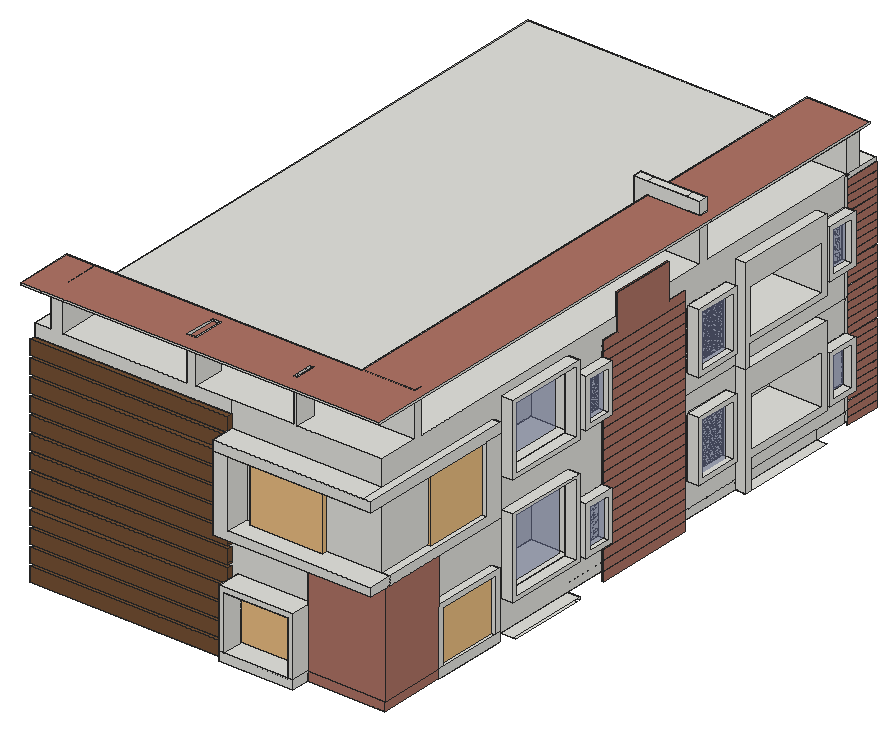
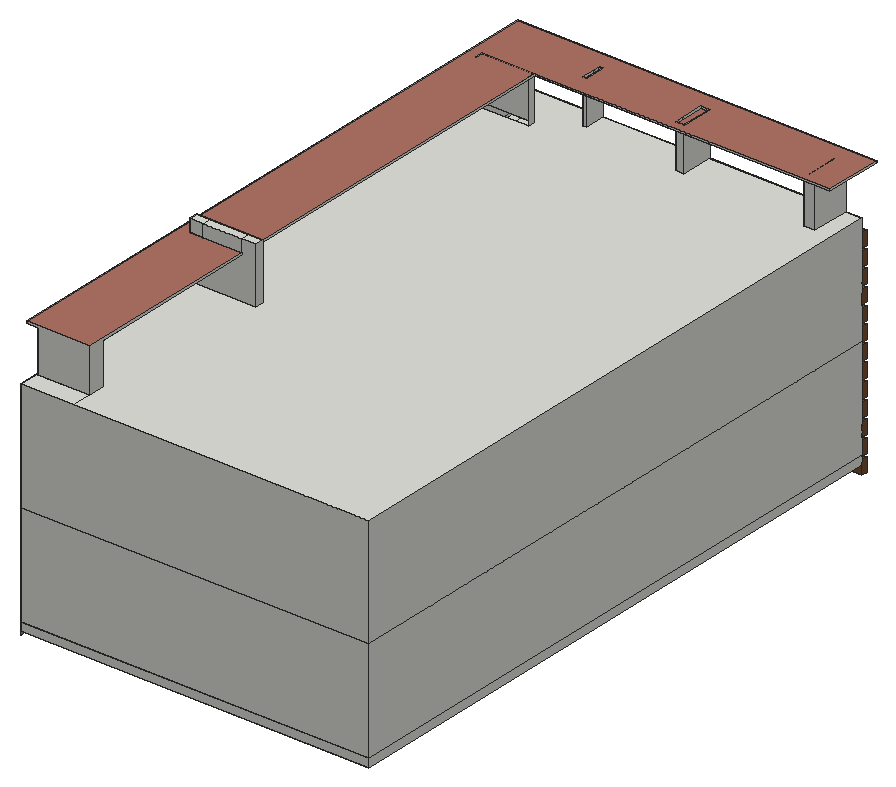
# SketchUp Ruby script. Lengths in inches.
U = 1.inch
M = Sketchup.active_model
def pt(a) = Geom::Point3d.new(a.map { |v| v * U })
def face(e, loops, mat)
  f = e.add_face(loops[0].map { |a| pt(a) })
  loops[1..].each { |l| e.add_face(l.map { |a| pt(a) }).erase! }
  f.material = f.back_material = mat if mat
  f
end
# faces: each face lists its corners as indices into pts; further lists are holes
def faces(e, pts, list, mat = nil) = list.each { |f| face(e, (f[0].is_a?(Array) ? f : [f]).map { |l| l.map { |i| pts[i] } }, mat) }
# xy, xz, yz: faces in a plane at the given z, y or x. An outline is a flat list of corners, or four numbers for a rectangle; further outlines are holes
def ring(l) = l.size == 4 ? [[l[0], l[1]], [l[2], l[1]], [l[2], l[3]], [l[0], l[3]]] : l.each_slice(2).to_a
def flat(e, list, mat, &to3) = list.each { |f| face(e, (f[0].is_a?(Array) ? f : [f]).map { |l| ring(l).map { |u, v| to3.(u, v) } }, mat) }
def xy(e, z, list, mat = nil) = flat(e, list, mat) { |x, y| [x, y, z] }
def xz(e, y, list, mat = nil) = flat(e, list, mat) { |x, z| [x, y, z] }
def yz(e, x, list, mat = nil) = flat(e, list, mat) { |y, z| [x, y, z] }
def lines(e, pts, list) = list.each { |a, b| e.add_line(pt(pts[a]), pt(pts[b])) }
# prism: a flat outline (further loops are holes) pulled along v
def prism(e, loops, v, mat = nil)
  f = face(e, loops, mat); d = Geom::Vector3d.new(v.map { |x| x * U })
  f.pushpull(f.normal.samedirection?(d) ? d.length : -d.length)
end
def box(e, o, s, mat = nil) = prism(e, [[o, [o[0] + s[0], o[1], o[2]], [o[0] + s[0], o[1] + s[1], o[2]], [o[0], o[1] + s[1], o[2]]]], [0, 0, s[2]], mat)
def at(x, y, z, deg = 0) = Geom::Transformation.translation(pt([x, y, z])) * Geom::Transformation.rotation(ORIGIN, Z_AXIS, deg.degrees)
def axes(o, x, y, z) = Geom::Transformation.new([*x, 0, *y, 0, *z, 0, *pt(o).to_a, 1])
def part(name) = M.definitions.add(name)
# library, detail: a bought-in or finely detailed component or shape, given as its bounding box
def library(name, o, s) = part(name).tap { |d| box(d.entities, o, s) }
def detail(e, o, s) = box(e.add_group.entities, o, s)
def put(e, d, t, mat = nil) = e.add_instance(d, t).tap { |i| i.material = mat if mat }
def group(e, t, mat = nil) = e.add_group.tap { |g| g.transformation = t; g.material = mat if mat }.entities
root = M.entities
M.materials.add("Artistic-Tile__Vetromarmi__Granada-Smoke-Glass-and-Stone-Wat").color = [172, 173, 170]
M.materials.add("[Sandstone]").color = [118, 81, 52]
M.materials.add("[Stone Flagstone Ashlar]").color = [175, 116, 102]
M.materials.add("[Translucent Glass Sky Reflection]").color = [126, 138, 183]
M.materials["[Translucent Glass Sky Reflection]"].alpha = 0.52
c1 = part("Group\#12")
prism(c1.entities,[[[0,67.07,0],[0,0,0],[0,0,12.125],[0,67.07,12.125],[0,139.8125,12.125],[0,139.8125,0]]],[2.5,0,0])
c2 = part("Group\#11")
prism(c2.entities,[[[271.64,0,19.53],[271.64,0,2.36],[271.64,0,0],[0,0,0],[0,0,19.53]]],[0,-6.9375,0])
c3 = part("Group\#13")
box(c3.entities,[0,0,0],[1.1875,48.5625,8.8125])
c4 = library("AS-120-mm\#2",[0,0,0],[88.21,4.72,72.97])
c5 = part("Group\#6")
xy(c5.entities,0,[[[0,0,45,67.3125],[6.42,6.42,38.58,60.9]],[6.42,6.42,38.58,60.9]])
xy(c5.entities,14.3125,[[[0,0,45,67.3125],[6.42,6.42,38.58,60.9]]])
xz(c5.entities,0,[[0,0,45,14.3125]])
xz(c5.entities,6.42,[[6.42,0,38.58,14.3125]])
xz(c5.entities,60.9,[[6.42,0,38.58,14.3125]])
xz(c5.entities,67.3125,[[0,0,45,14.3125]])
yz(c5.entities,0,[[0,0,67.3125,14.3125]])
yz(c5.entities,6.42,[[6.42,0,60.9,14.3125]])
yz(c5.entities,38.58,[[6.42,0,60.9,14.3125]])
yz(c5.entities,45,[[0,0,67.3125,14.3125]])
c6 = part("Group\#5")
xy(c6.entities,0,[[[0,0,66.75,83.5625],[5.83,5.83,60.92,77.73]],[5.83,5.83,60.92,77.73]])
xy(c6.entities,15.625,[[[0,0,66.75,83.5625],[5.83,5.83,60.92,77.73]]])
xz(c6.entities,0,[[0,0,66.75,15.625]])
xz(c6.entities,5.83,[[5.83,0,60.92,15.625]])
xz(c6.entities,77.73,[[5.83,0,60.92,15.625]])
xz(c6.entities,83.5625,[[0,0,66.75,15.625]])
yz(c6.entities,0,[[0,0,83.5625,15.625]])
yz(c6.entities,5.83,[[5.83,0,77.73,15.625]])
yz(c6.entities,60.92,[[5.83,0,77.73,15.625]])
yz(c6.entities,66.75,[[0,0,83.5625,15.625]])
c7 = part("Artistic-Tile__Vetromarmi__Granada-Smoke-Glass-and-Stone-Wat")
xy(c7.entities,0,[[0,0,24,24]],"[Translucent Glass Sky Reflection]")
c8 = library("AS-120-mm\#4",[0,0,0],[101.61,4.72,91.97])
c9 = library("AS-120-mm\#5",[0,0,0],[88.21,4.72,91.97])
xy(root,440.43,[[763.75,300.49,763.75,409.52,814.625,409.52,814.625,404.56,831,404.56,831,300.49]])
xy(root,443.8125,[[814.625,697.51,829.375,705.8]])
xy(root,444.1875,[[616.81,57.85,623.61,90.47],[623.61,57.85,711.82,90.47],[711.82,57.85,718.625,90.47],[718.69,83.16,814.625,83.16,814.625,174.47,824.98,174.47,824.98,181.28,814.625,181.28,814.625,271.67,824.98,271.67,824.98,278.47,814.625,278.47,814.625,939.04,336.5625,939.04,336.5625,90.47,718.69,90.47],[718.625,83.16,718.69,90.47],
  [814.625,83.16,824.98,174.47],[824.98,174.47,825.8125,181.28],[814.625,181.28,825.8125,271.67],[824.98,271.67,825.8125,278.47],[814.625,295.05,831,409.52],
  [814.625,697.51,828.9375,837.09]])
xy(root,456.1875,[[616.81,57.85,623.61,90.47],[623.61,57.85,711.82,90.47],[711.82,57.85,718.625,90.47],[718.69,83.16,718.69,90.47,336.5625,90.47,336.5625,939.04,814.625,939.04,814.625,409.52,763.75,409.52,763.75,295.05,814.625,295.05,814.625,278.47,825.8125,278.47,825.8125,271.67,814.625,271.67,814.625,181.28,825.8125,181.28,825.8125,174.47,814.625,174.47,814.625,83.16],[718.625,83.16,718.69,90.47],
  [814.625,83.16,824.98,174.47],[824.98,83.16,825.8125,174.47],[814.625,181.28,825.8125,271.67]])
xy(root,484.82,[[814.625,705.8,829.375,837.09]])
xy(root,487.375,[[814.625,295.05,831,409.52]])
xy(root,491.4375,[[763.75,295.05,814.625,300.49],[763.75,300.49,814.625,409.52],[814.625,300.49,831,404.56]])
xy(root,494.39,[[757.625,707.08,829.375,827.53]])
xy(root,528.43,[[814.625,181.28,825.8125,271.67]])
xy(root,531.09,[[623.61,57.85,711.82,90.47]])
xy(root,535.23,[[814.625,174.47,825.8125,278.47]])
xy(root,537.9,[[616.81,57.85,718.625,90.47]])
xy(root,562.5,[[757.625,707.08,829.375,827.53]])
xy(root,592.89,[[763.75,300.49,763.75,409.52,814.625,409.52,814.625,404.56,831,404.56,831,300.49]])
xy(root,596.25,[[814.625,295.05,831,409.52],[814.625,697.51,829.375,837.09]])
xy(root,596.375,[[763.75,295.05,814.625,409.52],[814.625,697.51,828.9375,704.26]])
xy(root,608.25,[[628.73,57.85,825.8125,90.47],[814.625,90.64,825.8125,257.14]])
xy(root,626.2,[[814.625,704.26,828.9375,837.09]])
xy(root,634.0625,[[755.875,705.37,828.9375,829.23]])
xy(root,638,[[814.625,295.05,831,409.52]])
xy(root,643.1875,[[763.75,295.05,814.625,300.49],[763.75,300.49,814.625,409.52],[814.625,300.49,831,404.56]])
xy(root,695.82,[[755.875,705.37,828.9375,829.23]])
xy(root,700.22,[[628.73,57.85,814.625,90.47],[814.625,57.85,825.8125,257.14]])
xy(root,713.98,[[608.2,57.85,814.625,90.47],[814.625,57.85,825.8125,280.55]])
xy(root,728.06,[[814.625,697.51,828.9375,837.09]])
xy(root,731.48,[[763.75,300.49,763.75,409.52,814.625,409.52,814.625,404.56,831,404.56,831,300.49]])
xy(root,735.98,[[814.625,295.05,831,409.52]])
xy(root,742.93,[[814.625,890.48,815.8125,939.04]])
xy(root,748.3125,[[336.5625,90.47,359.68,90.47,359.68,142.97,375.49,142.97,375.49,90.47,546.88,90.47,546.88,133.72,558.94,133.72,558.94,90.47,693.12,90.47,693.12,118.97,697.99,118.97,697.99,90.47,814.625,90.47,814.625,146.875,742.8125,146.875,742.8125,156.625,814.625,156.625,814.625,637.28,723.375,637.28,723.375,649.15,814.625,649.15,814.625,889.53,742.61,889.53,742.61,939.04,336.5625,939.04],[814.625,886.91,817.0625,890.48],[742.61,889.53,814.625,911.1],[814.625,890.48,815.8125,911.1],[742.61,911.1,815.8125,939.04]])
xy(root,805.9375,[[742.61,637.28,796.05,649.15],[814.625,637.28,814.625,649.15,742.61,649.15,742.61,889.53,829.6875,889.53,829.6875,637.28],[814.625,889.53,829.6875,911.1]])
xy(root,805.9375,[[336.5625,66.4,336.5625,145.68,742.61,145.68,742.61,637.28,829.6875,637.28,829.6875,66.4]],"[Stone Flagstone Ashlar]")
xy(root,807.1875,[[359.68,90.47,375.49,142.97]])
xy(root,808.4375,[[742.61,146.875,742.8125,156.625]])
xy(root,808.4375,[[[336.5625,66.4,829.6875,66.4,829.6875,911.1,742.61,911.1,742.61,156.625,742.8125,156.625,742.8125,146.875,742.61,146.875,742.61,145.68,336.5625,145.68],[546.88,90.47,558.94,133.72],[796.05,637.28,814.625,649.15],[693.12,90.47,697.99,118.97]]],"[Stone Flagstone Ashlar]")
xy(root,825.5625,[[723.375,637.28,742.61,649.15],[742.61,637.28,796.05,649.15],[796.05,637.28,814.625,649.15]])
xz(root,57.85,[[616.81,444.1875,718.625,456.1875],[616.81,456.1875,623.61,456.1875,623.61,531.09,711.82,531.09,711.82,456.1875,718.625,456.1875,718.625,537.9,616.81,537.9],[608.2,596.375,825.8125,596.375,825.8125,608.25,628.73,608.25,628.73,700.22,608.2,700.22],[608.2,700.22,825.8125,713.98]])
xz(root,66.4,[[336.5625,805.9375,829.6875,808.4375]])
xz(root,83.16,[[718.625,444.1875,718.69,456.1875]])
xz(root,83.16,[[718.69,444.1875,824.98,456.1875],[718.625,456.1875,825.8125,596.25]],"[Stone Flagstone Ashlar]")
xz(root,90.47,[[608.2,444.1875,616.81,456.1875],[718.625,444.1875,718.69,456.1875],[336.5625,456.1875,616.81,456.1875,616.81,537.9,718.625,537.9,718.625,596.25,336.5625,596.25],[623.61,456.1875,711.82,531.09],[336.5625,596.375,608.2,711.62],
  [814.625,596.375,825.8125,608.25],[628.73,608.25,814.625,700.22],[608.2,713.98,814.625,713.98,814.625,748.3125,697.99,748.3125,697.99,808.4375,693.12,808.4375,693.12,748.3125,608.2,748.3125],[336.5625,731.15,608.2,731.15,608.2,748.3125,558.94,748.3125,558.94,808.4375,546.88,808.4375,546.88,748.3125,375.49,748.3125,375.49,807.1875,359.68,807.1875,359.68,748.3125,336.5625,748.3125]])
xz(root,90.64,[[814.625,596.375,825.8125,608.25]])
xz(root,118.97,[[693.12,748.3125,697.99,808.4375]])
xz(root,133.72,[[546.88,748.3125,558.94,808.4375]])
xz(root,142.97,[[359.68,748.3125,375.49,807.1875]])
xz(root,145.68,[[336.5625,805.9375,742.61,808.4375]])
xz(root,146.875,[[742.8125,748.3125,814.625,808.4375]])
xz(root,174.47,[[824.98,444.1875,825.8125,456.1875],[814.625,535.23,825.8125,596.25]])
xz(root,181.28,[[814.625,456.1875,825.8125,528.43]])
xz(root,257.14,[[814.625,608.25,825.8125,700.22]])
xz(root,271.67,[[814.625,456.1875,825.8125,528.43]])
xz(root,278.47,[[814.625,444.1875,825.8125,456.1875],[814.625,456.1875,825.8125,535.23]])
xz(root,280.55,[[814.625,596.375,825.8125,700.22],[814.625,700.22,825.8125,713.98]])
xz(root,295.05,[[814.625,487.375,831,596.25],[763.75,596.25,814.625,596.375],[814.625,638,831,735.98]])
xz(root,300.49,[[763.75,491.4375,831,592.89],[763.75,643.1875,831,731.48]])
xz(root,404.56,[[814.625,491.4375,831,592.89],[814.625,643.1875,831,731.48]])
xz(root,409.52,[[763.75,440.43,814.625,444.1875],[814.625,440.43,831,444.1875],[814.625,487.375,831,592.89],[763.75,491.4375,814.625,592.89],[763.75,592.89,814.625,596.25],
  [814.625,592.89,831,596.25],[763.75,596.25,814.625,596.375],[814.625,638,831,731.48],[763.75,643.1875,814.625,731.48],[763.75,731.48,814.625,735.98],
  [814.625,731.48,831,735.98]])
xz(root,637.28,[[723.375,748.3125,814.625,748.3125,814.625,805.9375,796.05,805.9375,796.05,808.4375,814.625,808.4375,814.625,825.5625,723.375,825.5625],[796.05,805.9375,814.625,808.4375]])
xz(root,649.15,[[723.375,748.3125,723.375,825.5625,742.61,825.5625,742.61,805.9375,814.625,805.9375,814.625,748.3125],[742.61,805.9375,796.05,825.5625],[796.05,805.9375,814.625,808.4375],[796.05,808.4375,814.625,825.5625]])
xz(root,697.51,[[814.625,443.8125,828.9375,444.1875],[828.9375,443.8125,829.375,443.8125,829.375,596.25,814.625,596.25,814.625,444.1875,828.9375,444.1875],[814.625,596.375,828.9375,728.06]])
xz(root,704.26,[[814.625,596.375,828.9375,626.2]])
xz(root,705.37,[[755.875,634.0625,828.9375,695.82]])
xz(root,705.8,[[814.625,443.8125,829.375,484.82]])
xz(root,707.08,[[757.625,494.39,829.375,562.5]])
xz(root,827.53,[[757.625,494.39,829.375,562.5]])
xz(root,829.23,[[755.875,634.0625,828.9375,695.82]])
xz(root,837.09,[[814.625,484.82,829.375,596.25],[814.625,626.2,828.9375,728.06]])
xz(root,889.53,[[742.61,748.3125,814.625,805.9375]])
xz(root,890.48,[[814.625,742.93,815.8125,748.3125]])
xz(root,911.1,[[742.61,748.3125,742.61,808.4375,829.6875,808.4375,829.6875,805.9375,814.625,805.9375,814.625,748.3125]])
xz(root,939.04,[[336.5625,456.1875,814.625,596.25],[336.5625,596.375,814.625,748.3125],[814.625,742.93,815.8125,748.3125]])
yz(root,336.5625,[[90.47,456.1875,939.04,596.25],[90.47,596.375,939.04,748.3125],[66.4,805.9375,145.68,808.4375]])
yz(root,359.68,[[90.47,748.3125,142.97,807.1875]])
yz(root,375.49,[[90.47,748.3125,142.97,807.1875]])
yz(root,546.88,[[90.47,748.3125,133.72,808.4375]])
yz(root,558.94,[[90.47,748.3125,133.72,808.4375]])
yz(root,608.2,[[57.85,596.375,90.47,700.22],[57.85,700.22,90.47,713.98]])
yz(root,616.81,[[57.85,444.1875,90.47,456.1875],[57.85,456.1875,90.47,537.9]])
yz(root,623.61,[[57.85,456.1875,90.47,531.09]])
yz(root,628.73,[[57.85,608.25,90.47,700.22]])
yz(root,693.12,[[90.47,748.3125,118.97,808.4375]])
yz(root,697.99,[[90.47,748.3125,118.97,808.4375]])
yz(root,711.82,[[57.85,456.1875,90.47,531.09]])
yz(root,718.625,[[57.85,444.1875,83.16,456.1875],[83.16,444.1875,90.47,456.1875],[57.85,456.1875,83.16,537.9],[83.16,537.9,90.47,596.25]])
yz(root,718.69,[[83.16,444.1875,90.47,456.1875]])
yz(root,723.375,[[637.28,748.3125,649.15,825.5625]])
yz(root,742.61,[[889.53,748.3125,889.53,805.9375,649.15,805.9375,649.15,808.4375,911.1,808.4375,911.1,748.3125],[145.68,805.9375,637.28,808.4375],[637.28,805.9375,649.15,808.4375]])
yz(root,742.8125,[[146.875,748.3125,156.625,808.4375]])
yz(root,755.875,[[705.37,634.0625,829.23,695.82]])
yz(root,757.625,[[707.08,494.39,827.53,562.5]])
yz(root,763.75,[[295.05,456.1875,409.52,491.4375],[300.49,491.4375,409.52,592.89],[295.05,596.25,409.52,596.375],[295.05,596.375,409.52,643.1875],[300.49,643.1875,409.52,731.48]])
yz(root,796.05,[[637.28,805.9375,649.15,808.4375]])
yz(root,814.625,[[697.51,443.8125,705.8,444.1875],[[278.47,444.1875,468.48,444.1875,468.48,728.58,535.54,728.58,535.54,748.3125,156.625,748.3125,156.625,808.4375,146.875,808.4375,146.875,748.3125,90.47,748.3125,90.47,713.98,280.55,713.98,280.55,596.25,174.47,596.25,174.47,535.23,278.47,535.23],[295.05,487.375,409.52,596.375],[295.05,638,409.52,735.98]],[468.48,444.1875,535.54,456.1875],[535.54,444.1875,697.51,456.1875],[697.51,444.1875,705.8,456.1875],
  [705.8,444.1875,837.09,456.1875],[886.91,444.1875,890.48,456.1875],[181.28,456.1875,271.67,528.43],[468.48,456.1875,535.54,596.25],[535.54,456.1875,697.51,596.25],
  [705.8,456.1875,886.91,456.1875,886.91,596.25,837.09,596.25,837.09,484.82,705.8,484.82],[886.91,456.1875,890.48,596.25],[890.48,456.1875,939.04,596.25],[295.05,487.375,409.52,491.4375],[404.56,491.4375,409.52,592.89],
  [295.05,596.25,409.52,596.375],[468.48,596.25,535.54,596.375],[535.54,596.25,697.51,596.375],[697.51,596.25,837.09,596.375],[886.91,596.25,890.48,596.375],
  [90.47,596.375,90.64,596.375,90.64,608.25,257.14,608.25,257.14,700.22,90.47,700.22],[468.48,596.375,535.54,716.46],[535.54,596.375,697.51,596.375,697.51,728.06,837.09,728.06,837.09,626.2,704.26,626.2,704.26,596.375,886.91,596.375,886.91,748.3125,649.15,748.3125,649.15,805.9375,637.28,805.9375,637.28,748.3125,535.54,748.3125,535.54,728.58,608.29,728.58,608.29,716.46,535.54,716.46],[886.91,596.375,890.48,748.3125],[890.48,596.375,939.04,733],
  [295.05,638,409.52,643.1875],[404.56,643.1875,409.52,731.48],[890.48,741.8125,939.04,742.93],[889.53,748.3125,911.1,805.9375],[637.28,805.9375,649.15,808.4375],
  [637.28,808.4375,649.15,825.5625]])
yz(root,815.8125,[[890.48,742.93,939.04,748.3125]])
yz(root,824.98,[[83.16,444.1875,174.47,456.1875]],"[Stone Flagstone Ashlar]")
yz(root,825.8125,[[174.47,444.1875,278.47,456.1875],[174.47,456.1875,181.28,456.1875,181.28,528.43,271.67,528.43,271.67,456.1875,278.47,456.1875,278.47,535.23,174.47,535.23],[57.85,596.375,90.47,608.25],[90.64,596.375,280.55,596.375,280.55,700.22,257.14,700.22,257.14,608.25,90.64,608.25],[57.85,700.22,280.55,713.98]])
yz(root,825.8125,[[83.16,456.1875,174.47,596.25]],"[Stone Flagstone Ashlar]")
yz(root,828.9375,[[697.51,596.375,704.26,596.375,704.26,626.2,837.09,626.2,837.09,718.19,705.37,718.19,705.37,695.82,829.23,695.82,829.23,634.0625,705.37,634.0625,705.37,718.19,837.09,718.19,837.09,728.06,697.51,728.06]])
yz(root,829.375,[[[697.51,443.8125,705.8,443.8125,705.8,484.82,837.09,484.82,837.09,596.25,697.51,596.25],[707.08,494.39,827.53,562.5]]])
yz(root,829.6875,[[66.4,805.9375,637.28,808.4375],[637.28,805.9375,911.1,808.4375]])
yz(root,831,[[[295.05,487.375,409.52,596.25],[300.49,491.4375,404.56,592.89]],[[295.05,638,409.52,735.98],[300.49,643.1875,404.56,731.48]]])
p = [[608.2,90.47,596.25],[608.2,90.47,596.375],[817.125,493.42,728.58],[814.625,493.42,728.58],[817.125,580.72,728.58],[814.625,580.72,728.58]]
lines(root,p,[[0,1],[2,3],[4,5]])
put(root,c1,at(814.625,468.48,431.64),"[Stone Flagstone Ashlar]")
put(root,c2,at(336.5625,90.47,431.87),"[Sandstone]")
put(root,c3,at(814.625,890.48,439.375),"[Stone Flagstone Ashlar]")
g1 = group(root,at(336.5625,690.47,444.1875))
box(g1,[0,-600,0],[478.0625,848.5625,12])
put(root,c1,at(814.625,468.48,445.21),"[Stone Flagstone Ashlar]")
put(root,c3,at(814.625,890.48,449.5),"[Stone Flagstone Ashlar]")
put(root,c2,at(336.5625,90.47,455.18),"[Sandstone]")
put(root,c4,at(815.4375,271.67,455.46,-90))
put(root,c4,at(623.61,85.95,458.12))
put(root,c1,at(814.625,468.48,458.77),"[Stone Flagstone Ashlar]")
put(root,c3,at(814.625,890.48,459.625),"[Stone Flagstone Ashlar]")
put(root,c3,at(814.625,890.48,469.75),"[Stone Flagstone Ashlar]")
put(root,c1,at(814.625,468.48,472.33),"[Stone Flagstone Ashlar]")
put(root,c2,at(336.5625,90.47,478.49),"[Sandstone]")
put(root,c3,at(814.625,890.48,479.875),"[Stone Flagstone Ashlar]")
g2 = group(root,at(814.625,423.48,484.47))
xy(g2,0,[[0,0,14.3125,45]])
xy(g2,6.42,[[0,6.42,14.3125,38.58]])
xy(g2,60.9,[[0,6.42,14.3125,38.58]])
xy(g2,67.3125,[[0,0,14.3125,45]])
xz(g2,0,[[0,0,14.3125,67.3125]])
xz(g2,6.42,[[0,6.42,14.3125,60.9]])
xz(g2,38.58,[[0,6.42,14.3125,60.9]])
xz(g2,45,[[0,0,14.3125,67.3125]])
yz(g2,0,[[[0,0,45,67.3125],[6.42,6.42,38.58,60.9]],[6.42,6.42,38.58,60.9]])
yz(g2,14.3125,[[[0,0,45,67.3125],[6.42,6.42,38.58,60.9]]])
put(root,c1,at(814.625,468.48,485.89),"[Stone Flagstone Ashlar]")
put(root,c5,axes([814.625,841.91,487.29],[0,1,0],[0,0,1],[1,0,0]))
put(root,c3,at(814.625,890.48,490),"[Stone Flagstone Ashlar]")
put(root,c6,axes([814.625,615.15,490.8],[0,1,0],[0,0,1],[1,0,0]))
put(root,c7,axes([823.9375,462.06,545.37],[0,-1.33,0],[0,0,-2.26992],[1,0,0]))
put(root,c7,axes([808.6875,404.56,592.89],[0,-4.33639,0],[0,0,-4.22736],[1,0,0]))
put(root,c7,axes([822.4375,672.37,566.21],[0,-2.1413,0],[0,0,-3.0449],[1,0,0]))
put(root,c7,axes([817.8125,880.25,548.18],[0,-1.33,0],[0,0,-2.26992],[1,0,0]))
put(root,c1,at(814.625,468.48,499.46),"[Stone Flagstone Ashlar]")
put(root,c3,at(814.625,890.48,500.125),"[Stone Flagstone Ashlar]")
put(root,c2,at(336.5625,90.47,501.8),"[Sandstone]")
put(root,c3,at(814.625,890.48,510.25),"[Stone Flagstone Ashlar]")
put(root,c1,at(814.625,468.48,513.02),"[Stone Flagstone Ashlar]")
put(root,c3,at(814.625,890.48,520.375),"[Stone Flagstone Ashlar]")
put(root,c2,at(336.5625,90.47,525.12),"[Sandstone]")
put(root,c1,at(814.625,468.48,526.58),"[Stone Flagstone Ashlar]")
put(root,c3,at(814.625,890.48,530.5),"[Stone Flagstone Ashlar]")
put(root,c1,at(814.625,468.48,540.14),"[Stone Flagstone Ashlar]")
put(root,c3,at(814.625,890.48,540.625),"[Stone Flagstone Ashlar]")
put(root,c2,at(336.5625,90.47,548.43),"[Sandstone]")
put(root,c3,at(814.625,890.48,550.75),"[Stone Flagstone Ashlar]")
put(root,c1,at(814.625,468.48,553.71),"[Stone Flagstone Ashlar]")
put(root,c3,at(814.625,890.48,560.875),"[Stone Flagstone Ashlar]")
put(root,c1,at(814.625,468.48,567.27),"[Stone Flagstone Ashlar]")
put(root,c3,at(814.625,890.48,571),"[Stone Flagstone Ashlar]")
put(root,c2,at(336.5625,90.47,571.74),"[Sandstone]")
put(root,c1,at(814.625,468.48,580.83),"[Stone Flagstone Ashlar]")
put(root,c3,at(814.625,890.48,581.125),"[Stone Flagstone Ashlar]")
put(root,c3,at(814.625,890.48,591.25),"[Stone Flagstone Ashlar]")
put(root,c1,at(814.625,468.48,594.39),"[Stone Flagstone Ashlar]")
put(root,c2,at(336.5625,90.47,595.05),"[Sandstone]")
put(root,c3,at(814.625,890.48,601.375),"[Stone Flagstone Ashlar]")
put(root,c1,at(814.625,468.48,607.96),"[Stone Flagstone Ashlar]")
put(root,c8,at(638.25,83.22,608.25))
put(root,c9,at(814.09,257.14,608.25,-90))
put(root,c3,at(814.625,890.48,611.5),"[Stone Flagstone Ashlar]")
put(root,c2,at(336.5625,90.47,618.37),"[Sandstone]")
put(root,c1,at(814.625,468.48,621.52),"[Stone Flagstone Ashlar]")
put(root,c3,at(814.625,890.48,621.625),"[Stone Flagstone Ashlar]")
put(root,c6,axes([814.625,615.15,623.93],[0,1,0],[0,0,1],[1,0,0]))
put(root,c7,axes([822.4375,672.37,702.84],[0,-2.1413,0],[0,0,-3.0449],[1,0,0]))
put(root,c3,at(814.625,890.48,631.75),"[Stone Flagstone Ashlar]")
put(root,c1,at(814.625,468.48,635.08),"[Stone Flagstone Ashlar]")
put(root,c5,axes([814.625,423.48,641.54],[0,1,0],[0,0,1],[1,0,0]))
put(root,c5,axes([814.625,841.91,641.54],[0,1,0],[0,0,1],[1,0,0]))
put(root,c2,at(336.5625,90.47,641.68),"[Sandstone]")
put(root,c3,at(814.625,890.48,641.875),"[Stone Flagstone Ashlar]")
put(root,c7,axes([802.08,404.56,731.48],[0,-4.33639,0],[0,0,-3.67875],[1,0,0]))
put(root,c7,axes([822.9375,462.06,702.43],[0,-1.33,0],[0,0,-2.26992],[1,0,0]))
put(root,c7,axes([820.9375,880.25,702.43],[0,-1.33,0],[0,0,-2.26992],[1,0,0]))
put(root,c1,at(814.625,468.48,648.64),"[Stone Flagstone Ashlar]")
put(root,c3,at(814.625,890.48,652),"[Stone Flagstone Ashlar]")
put(root,c3,at(814.625,890.48,662.125),"[Stone Flagstone Ashlar]")
put(root,c1,at(814.625,468.48,662.21),"[Stone Flagstone Ashlar]")
put(root,c2,at(336.5625,90.47,664.99),"[Sandstone]")
put(root,c3,at(814.625,890.48,672.25),"[Stone Flagstone Ashlar]")
put(root,c1,at(814.625,468.48,675.77),"[Stone Flagstone Ashlar]")
put(root,c3,at(814.625,890.48,682.375),"[Stone Flagstone Ashlar]")
put(root,c2,at(336.5625,90.47,688.3),"[Sandstone]")
put(root,c1,at(814.625,468.48,689.33),"[Stone Flagstone Ashlar]")
put(root,c3,at(814.625,890.48,692.5),"[Stone Flagstone Ashlar]")
put(root,c3,at(814.625,890.48,702.625),"[Stone Flagstone Ashlar]")
put(root,c1,at(814.625,468.48,702.89),"[Stone Flagstone Ashlar]")
put(root,c2,at(336.5625,90.47,711.62),"[Sandstone]")
put(root,c3,at(814.625,890.48,712.75),"[Stone Flagstone Ashlar]")
g3 = group(root,at(814.625,468.48,716.46),"[Stone Flagstone Ashlar]")
prism(g3,[[[0,67.07,0],[0,0,0],[0,0,12.125],[0,24.94,12.125],[0,24.94,60.54],[0,67.07,60.54],[0,112.29,60.54],[0,112.29,12.125],[0,139.8125,12.125],[0,139.8125,0]]],[2.5,0,0])
put(root,c3,at(814.625,890.48,722.875),"[Stone Flagstone Ashlar]")
put(root,c3,at(814.625,890.48,733),"[Stone Flagstone Ashlar]")
